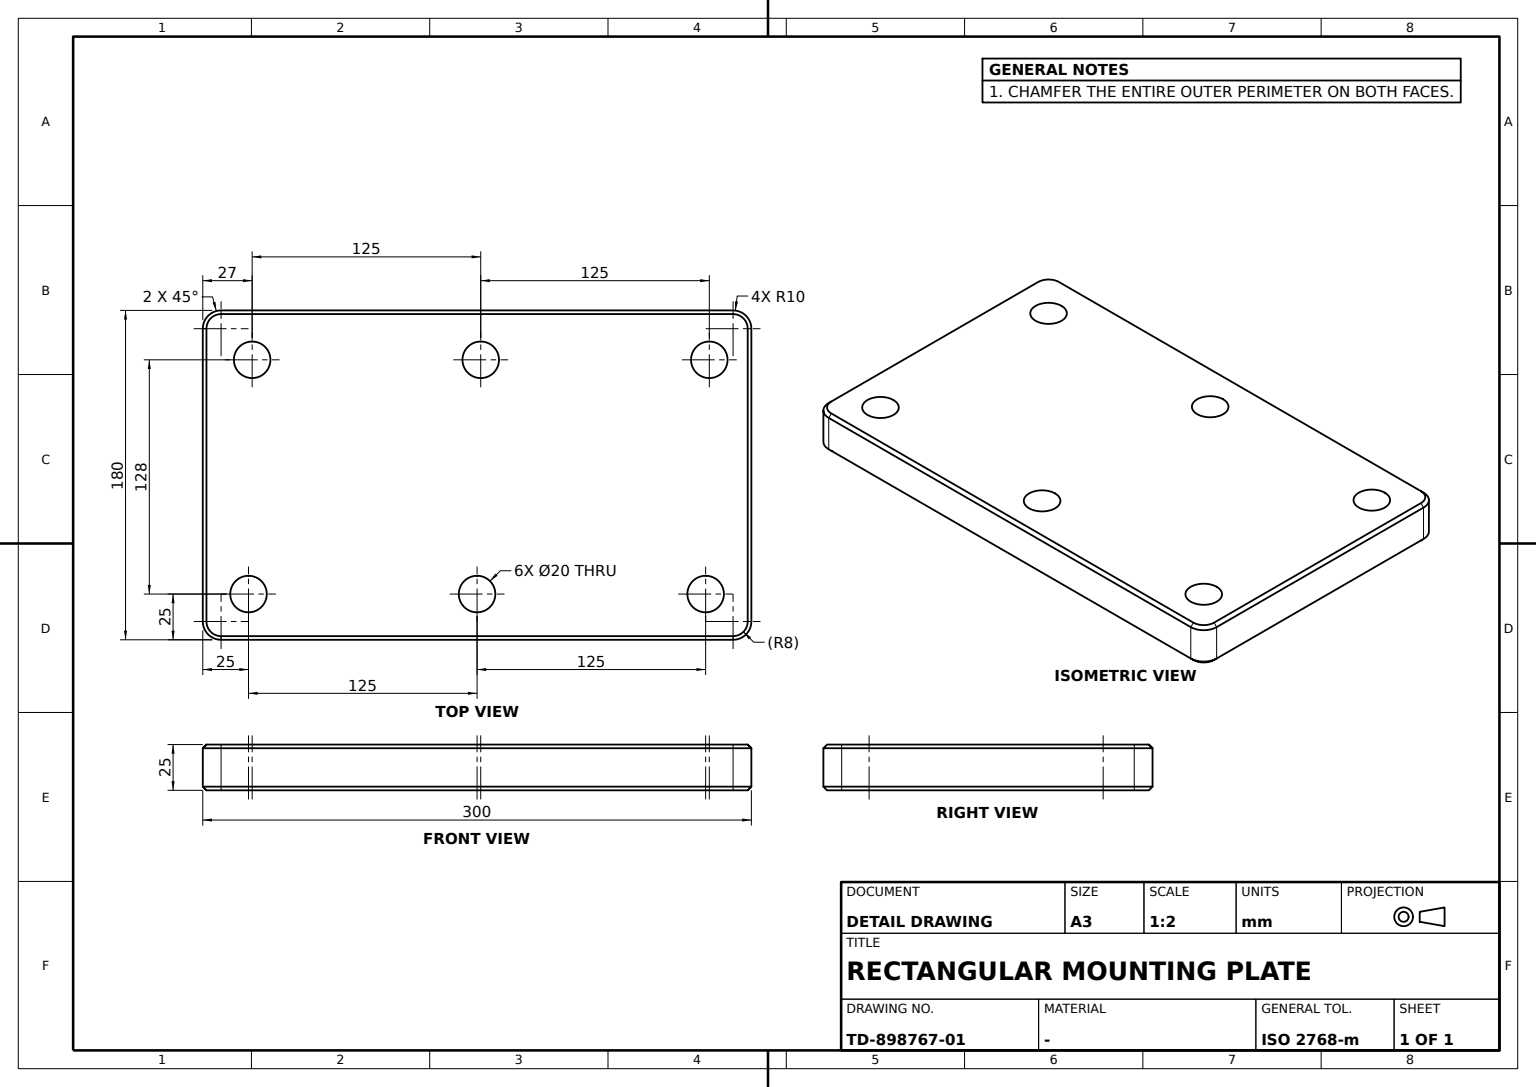
ISO-10303-21;
HEADER;
FILE_DESCRIPTION((''),'2;1');
FILE_NAME('','',(''),(''),'','','');
FILE_SCHEMA(('AUTOMOTIVE_DESIGN'));
ENDSEC;
DATA;
#1=APPLICATION_CONTEXT('');
#2=PRODUCT_CONTEXT('',#1,'mechanical');
#3=PRODUCT('','','',(#2));
#4=PRODUCT_DEFINITION_FORMATION('','',#3);
#5=PRODUCT_DEFINITION_CONTEXT('',#1,'design');
#6=PRODUCT_DEFINITION('','',#4,#5);
#7=PRODUCT_DEFINITION_SHAPE('','',#6);
#8=(LENGTH_UNIT()NAMED_UNIT(*)SI_UNIT(.MILLI.,.METRE.));
#9=(NAMED_UNIT(*)PLANE_ANGLE_UNIT()SI_UNIT($,.RADIAN.));
#10=(NAMED_UNIT(*)SI_UNIT($,.STERADIAN.)SOLID_ANGLE_UNIT());
#11=UNCERTAINTY_MEASURE_WITH_UNIT(LENGTH_MEASURE(0.005),#8,'distance_accuracy_value','');
#12=(GEOMETRIC_REPRESENTATION_CONTEXT(3)GLOBAL_UNCERTAINTY_ASSIGNED_CONTEXT((#11))GLOBAL_UNIT_ASSIGNED_CONTEXT((#8,#9,#10))REPRESENTATION_CONTEXT('',''));
#13=CARTESIAN_POINT('',(-73.,127.,12.5));
#14=VERTEX_POINT('',#13);
#15=CARTESIAN_POINT('',(-63.,127.,12.5));
#16=DIRECTION('',(0.,0.,-1.));
#17=DIRECTION('',(-1.,0.,0.));
#18=AXIS2_PLACEMENT_3D('',#15,#16,#17);
#19=CIRCLE('',#18,10.);
#20=EDGE_CURVE('',#14,#14,#19,.T.);
#21=ORIENTED_EDGE('',*,*,#20,.F.);
#22=EDGE_LOOP('',(#21));
#23=FACE_BOUND('',#22,.T.);
#24=CARTESIAN_POINT('',(-73.,127.,-12.5));
#25=VERTEX_POINT('',#24);
#26=CARTESIAN_POINT('',(-63.,127.,-12.5));
#27=AXIS2_PLACEMENT_3D('',#26,#16,#17);
#28=CIRCLE('',#27,10.);
#29=EDGE_CURVE('',#25,#25,#28,.T.);
#30=ORIENTED_EDGE('',*,*,#29,.T.);
#31=EDGE_LOOP('',(#30));
#32=FACE_BOUND('',#31,.T.);
#33=CARTESIAN_POINT('',(-63.,127.,12.4));
#34=DIRECTION('',(1.,0.,0.));
#35=AXIS2_PLACEMENT_3D('',#33,#16,#34);
#36=CYLINDRICAL_SURFACE('',#35,10.);
#37=ADVANCED_FACE('',(#23,#32),#36,.F.);
#38=CARTESIAN_POINT('',(80.,148.,-12.5));
#39=VERTEX_POINT('',#38);
#40=CARTESIAN_POINT('',(80.,150.,-10.5));
#41=VERTEX_POINT('',#40);
#42=CARTESIAN_POINT('',(80.,140.,-20.5));
#43=DIRECTION('',(0.,0.707106781,0.707106781));
#44=VECTOR('',#43,1000.);
#45=LINE('',#42,#44);
#46=EDGE_CURVE('',#39,#41,#45,.T.);
#47=ORIENTED_EDGE('',*,*,#46,.F.);
#48=CARTESIAN_POINT('',(-80.,148.,-12.5));
#49=VERTEX_POINT('',#48);
#50=CARTESIAN_POINT('',(-126.,148.,-12.5));
#51=VECTOR('',#34,1000.);
#52=LINE('',#50,#51);
#53=EDGE_CURVE('',#49,#39,#52,.T.);
#54=ORIENTED_EDGE('',*,*,#53,.F.);
#55=CARTESIAN_POINT('',(-80.,150.,-10.5));
#56=VERTEX_POINT('',#55);
#57=CARTESIAN_POINT('',(-80.,140.,-20.5));
#58=LINE('',#57,#44);
#59=EDGE_CURVE('',#49,#56,#58,.T.);
#60=ORIENTED_EDGE('',*,*,#59,.T.);
#61=CARTESIAN_POINT('',(-90.,150.,-10.5));
#62=LINE('',#61,#51);
#63=EDGE_CURVE('',#56,#41,#62,.T.);
#64=ORIENTED_EDGE('',*,*,#63,.T.);
#65=EDGE_LOOP('',(#47,#54,#60,#64));
#66=FACE_BOUND('',#65,.T.);
#67=DIRECTION('',(0.,-0.707106781,0.707106781));
#68=AXIS2_PLACEMENT_3D('',#50,#67,#34);
#69=PLANE('',#68);
#70=ADVANCED_FACE('',(#66),#69,.F.);
#71=CARTESIAN_POINT('',(-80.,150.,10.5));
#72=VERTEX_POINT('',#71);
#73=CARTESIAN_POINT('',(-80.,150.,0.));
#74=VECTOR('',#16,1000.);
#75=LINE('',#73,#74);
#76=EDGE_CURVE('',#72,#56,#75,.T.);
#77=ORIENTED_EDGE('',*,*,#76,.F.);
#78=CARTESIAN_POINT('',(80.,150.,10.5));
#79=VERTEX_POINT('',#78);
#80=CARTESIAN_POINT('',(-90.,150.,10.5));
#81=LINE('',#80,#51);
#82=EDGE_CURVE('',#72,#79,#81,.T.);
#83=ORIENTED_EDGE('',*,*,#82,.T.);
#84=CARTESIAN_POINT('',(80.,150.,0.));
#85=LINE('',#84,#74);
#86=EDGE_CURVE('',#79,#41,#85,.T.);
#87=ORIENTED_EDGE('',*,*,#86,.T.);
#88=ORIENTED_EDGE('',*,*,#63,.F.);
#89=EDGE_LOOP('',(#77,#83,#87,#88));
#90=FACE_BOUND('',#89,.T.);
#91=CARTESIAN_POINT('',(-90.,150.,0.));
#92=DIRECTION('',(0.,1.,0.));
#93=AXIS2_PLACEMENT_3D('',#91,#92,#34);
#94=PLANE('',#93);
#95=ADVANCED_FACE('',(#90),#94,.T.);
#96=CARTESIAN_POINT('',(-80.,-148.,-12.5));
#97=VERTEX_POINT('',#96);
#98=CARTESIAN_POINT('',(-80.,-150.,-10.5));
#99=VERTEX_POINT('',#98);
#100=CARTESIAN_POINT('',(-80.,-140.,-20.5));
#101=VECTOR('',#67,1000.);
#102=LINE('',#100,#101);
#103=EDGE_CURVE('',#97,#99,#102,.T.);
#104=ORIENTED_EDGE('',*,*,#103,.F.);
#105=CARTESIAN_POINT('',(80.,-148.,-12.5));
#106=VERTEX_POINT('',#105);
#107=CARTESIAN_POINT('',(126.,-148.,-12.5));
#108=VECTOR('',#17,1000.);
#109=LINE('',#107,#108);
#110=EDGE_CURVE('',#106,#97,#109,.T.);
#111=ORIENTED_EDGE('',*,*,#110,.F.);
#112=CARTESIAN_POINT('',(80.,-150.,-10.5));
#113=VERTEX_POINT('',#112);
#114=CARTESIAN_POINT('',(80.,-140.,-20.5));
#115=LINE('',#114,#101);
#116=EDGE_CURVE('',#106,#113,#115,.T.);
#117=ORIENTED_EDGE('',*,*,#116,.T.);
#118=CARTESIAN_POINT('',(90.,-150.,-10.5));
#119=LINE('',#118,#108);
#120=EDGE_CURVE('',#113,#99,#119,.T.);
#121=ORIENTED_EDGE('',*,*,#120,.T.);
#122=EDGE_LOOP('',(#104,#111,#117,#121));
#123=FACE_BOUND('',#122,.T.);
#124=AXIS2_PLACEMENT_3D('',#107,#43,#17);
#125=PLANE('',#124);
#126=ADVANCED_FACE('',(#123),#125,.F.);
#127=CARTESIAN_POINT('',(55.,0.,-12.5));
#128=VERTEX_POINT('',#127);
#129=CARTESIAN_POINT('',(65.,0.,-12.5));
#130=AXIS2_PLACEMENT_3D('',#129,#16,#17);
#131=CIRCLE('',#130,10.);
#132=EDGE_CURVE('',#128,#128,#131,.T.);
#133=ORIENTED_EDGE('',*,*,#132,.T.);
#134=EDGE_LOOP('',(#133));
#135=FACE_BOUND('',#134,.T.);
#136=CARTESIAN_POINT('',(55.,0.,12.5));
#137=VERTEX_POINT('',#136);
#138=CARTESIAN_POINT('',(65.,0.,12.5));
#139=AXIS2_PLACEMENT_3D('',#138,#16,#17);
#140=CIRCLE('',#139,10.);
#141=EDGE_CURVE('',#137,#137,#140,.T.);
#142=ORIENTED_EDGE('',*,*,#141,.F.);
#143=EDGE_LOOP('',(#142));
#144=FACE_BOUND('',#143,.T.);
#145=CARTESIAN_POINT('',(65.,0.,12.4));
#146=AXIS2_PLACEMENT_3D('',#145,#16,#34);
#147=CYLINDRICAL_SURFACE('',#146,10.);
#148=ADVANCED_FACE('',(#135,#144),#147,.F.);
#149=CARTESIAN_POINT('',(-80.,-150.,10.5));
#150=VERTEX_POINT('',#149);
#151=CARTESIAN_POINT('',(-90.,-140.,10.5));
#152=VERTEX_POINT('',#151);
#153=CARTESIAN_POINT('',(-80.,-140.,10.5));
#154=AXIS2_PLACEMENT_3D('',#153,#16,#17);
#155=CIRCLE('',#154,10.);
#156=EDGE_CURVE('',#150,#152,#155,.T.);
#157=ORIENTED_EDGE('',*,*,#156,.F.);
#158=CARTESIAN_POINT('',(-80.,-148.,12.5));
#159=VERTEX_POINT('',#158);
#160=CARTESIAN_POINT('',(-80.,-140.,20.5));
#161=DIRECTION('',(0.,-0.707106781,-0.707106781));
#162=VECTOR('',#161,1000.);
#163=LINE('',#160,#162);
#164=EDGE_CURVE('',#159,#150,#163,.T.);
#165=ORIENTED_EDGE('',*,*,#164,.F.);
#166=CARTESIAN_POINT('',(-88.,-140.,12.5));
#167=VERTEX_POINT('',#166);
#168=CARTESIAN_POINT('',(-80.,-140.,12.5));
#169=AXIS2_PLACEMENT_3D('',#168,#16,#17);
#170=CIRCLE('',#169,8.);
#171=EDGE_CURVE('',#159,#167,#170,.T.);
#172=ORIENTED_EDGE('',*,*,#171,.T.);
#173=DIRECTION('',(-0.707106781,0.,-0.707106781));
#174=VECTOR('',#173,1000.);
#175=LINE('',#160,#174);
#176=EDGE_CURVE('',#167,#152,#175,.T.);
#177=ORIENTED_EDGE('',*,*,#176,.T.);
#178=EDGE_LOOP('',(#157,#165,#172,#177));
#179=FACE_BOUND('',#178,.T.);
#180=DIRECTION('',(0.459989449,-0.887924381,0.));
#181=AXIS2_PLACEMENT_3D('',#160,#16,#180);
#182=CONICAL_SURFACE('',#181,0.,0.785398163);
#183=ADVANCED_FACE('',(#179),#182,.T.);
#184=CARTESIAN_POINT('',(-80.,-150.,0.));
#185=LINE('',#184,#74);
#186=EDGE_CURVE('',#150,#99,#185,.T.);
#187=ORIENTED_EDGE('',*,*,#186,.T.);
#188=ORIENTED_EDGE('',*,*,#120,.F.);
#189=CARTESIAN_POINT('',(80.,-150.,10.5));
#190=VERTEX_POINT('',#189);
#191=CARTESIAN_POINT('',(80.,-150.,0.));
#192=LINE('',#191,#74);
#193=EDGE_CURVE('',#190,#113,#192,.T.);
#194=ORIENTED_EDGE('',*,*,#193,.F.);
#195=CARTESIAN_POINT('',(90.,-150.,10.5));
#196=LINE('',#195,#108);
#197=EDGE_CURVE('',#190,#150,#196,.T.);
#198=ORIENTED_EDGE('',*,*,#197,.T.);
#199=EDGE_LOOP('',(#187,#188,#194,#198));
#200=FACE_BOUND('',#199,.T.);
#201=CARTESIAN_POINT('',(90.,-150.,0.));
#202=DIRECTION('',(0.,-1.,0.));
#203=AXIS2_PLACEMENT_3D('',#201,#202,#17);
#204=PLANE('',#203);
#205=ADVANCED_FACE('',(#200),#204,.T.);
#206=CARTESIAN_POINT('',(90.,140.,10.5));
#207=VERTEX_POINT('',#206);
#208=CARTESIAN_POINT('',(90.,140.,-10.5));
#209=VERTEX_POINT('',#208);
#210=CARTESIAN_POINT('',(90.,140.,0.));
#211=LINE('',#210,#74);
#212=EDGE_CURVE('',#207,#209,#211,.T.);
#213=ORIENTED_EDGE('',*,*,#212,.F.);
#214=CARTESIAN_POINT('',(90.,-140.,10.5));
#215=VERTEX_POINT('',#214);
#216=CARTESIAN_POINT('',(90.,-210.,10.5));
#217=VECTOR('',#92,1000.);
#218=LINE('',#216,#217);
#219=EDGE_CURVE('',#215,#207,#218,.T.);
#220=ORIENTED_EDGE('',*,*,#219,.F.);
#221=CARTESIAN_POINT('',(90.,-140.,-10.5));
#222=VERTEX_POINT('',#221);
#223=CARTESIAN_POINT('',(90.,-140.,0.));
#224=LINE('',#223,#74);
#225=EDGE_CURVE('',#215,#222,#224,.T.);
#226=ORIENTED_EDGE('',*,*,#225,.T.);
#227=CARTESIAN_POINT('',(90.,-210.,-10.5));
#228=LINE('',#227,#217);
#229=EDGE_CURVE('',#222,#209,#228,.T.);
#230=ORIENTED_EDGE('',*,*,#229,.T.);
#231=EDGE_LOOP('',(#213,#220,#226,#230));
#232=FACE_BOUND('',#231,.T.);
#233=AXIS2_PLACEMENT_3D('',#201,#17,#92);
#234=PLANE('',#233);
#235=ADVANCED_FACE('',(#232),#234,.F.);
#236=CARTESIAN_POINT('',(-90.,140.,-10.5));
#237=VERTEX_POINT('',#236);
#238=CARTESIAN_POINT('',(-90.,-140.,-10.5));
#239=VERTEX_POINT('',#238);
#240=CARTESIAN_POINT('',(-90.,210.,-10.5));
#241=VECTOR('',#202,1000.);
#242=LINE('',#240,#241);
#243=EDGE_CURVE('',#237,#239,#242,.T.);
#244=ORIENTED_EDGE('',*,*,#243,.F.);
#245=CARTESIAN_POINT('',(-88.,140.,-12.5));
#246=VERTEX_POINT('',#245);
#247=DIRECTION('',(-0.707106781,0.,0.707106781));
#248=VECTOR('',#247,1000.);
#249=LINE('',#57,#248);
#250=EDGE_CURVE('',#246,#237,#249,.T.);
#251=ORIENTED_EDGE('',*,*,#250,.F.);
#252=CARTESIAN_POINT('',(-88.,-140.,-12.5));
#253=VERTEX_POINT('',#252);
#254=CARTESIAN_POINT('',(-88.,210.,-12.5));
#255=LINE('',#254,#241);
#256=EDGE_CURVE('',#246,#253,#255,.T.);
#257=ORIENTED_EDGE('',*,*,#256,.T.);
#258=LINE('',#100,#248);
#259=EDGE_CURVE('',#253,#239,#258,.T.);
#260=ORIENTED_EDGE('',*,*,#259,.T.);
#261=EDGE_LOOP('',(#244,#251,#257,#260));
#262=FACE_BOUND('',#261,.T.);
#263=AXIS2_PLACEMENT_3D('',#254,#173,#202);
#264=PLANE('',#263);
#265=ADVANCED_FACE('',(#262),#264,.T.);
#266=CARTESIAN_POINT('',(88.,-140.,12.5));
#267=VERTEX_POINT('',#266);
#268=CARTESIAN_POINT('',(80.,-148.,12.5));
#269=VERTEX_POINT('',#268);
#270=CARTESIAN_POINT('',(80.,-140.,12.5));
#271=AXIS2_PLACEMENT_3D('',#270,#16,#17);
#272=CIRCLE('',#271,8.);
#273=EDGE_CURVE('',#267,#269,#272,.T.);
#274=ORIENTED_EDGE('',*,*,#273,.T.);
#275=CARTESIAN_POINT('',(80.,-140.,20.5));
#276=LINE('',#275,#162);
#277=EDGE_CURVE('',#269,#190,#276,.T.);
#278=ORIENTED_EDGE('',*,*,#277,.T.);
#279=CARTESIAN_POINT('',(80.,-140.,10.5));
#280=AXIS2_PLACEMENT_3D('',#279,#16,#92);
#281=CIRCLE('',#280,10.);
#282=EDGE_CURVE('',#215,#190,#281,.T.);
#283=ORIENTED_EDGE('',*,*,#282,.F.);
#284=DIRECTION('',(0.707106781,0.,-0.707106781));
#285=VECTOR('',#284,1000.);
#286=LINE('',#275,#285);
#287=EDGE_CURVE('',#267,#215,#286,.T.);
#288=ORIENTED_EDGE('',*,*,#287,.F.);
#289=EDGE_LOOP('',(#274,#278,#283,#288));
#290=FACE_BOUND('',#289,.T.);
#291=DIRECTION('',(0.887924381,0.459989449,0.));
#292=AXIS2_PLACEMENT_3D('',#275,#16,#291);
#293=CONICAL_SURFACE('',#292,0.,0.785398163);
#294=ADVANCED_FACE('',(#290),#293,.T.);
#295=ORIENTED_EDGE('',*,*,#116,.F.);
#296=CARTESIAN_POINT('',(88.,-140.,-12.5));
#297=VERTEX_POINT('',#296);
#298=CARTESIAN_POINT('',(80.,-140.,-12.5));
#299=AXIS2_PLACEMENT_3D('',#298,#16,#17);
#300=CIRCLE('',#299,8.);
#301=EDGE_CURVE('',#297,#106,#300,.T.);
#302=ORIENTED_EDGE('',*,*,#301,.F.);
#303=DIRECTION('',(0.707106781,0.,0.707106781));
#304=VECTOR('',#303,1000.);
#305=LINE('',#114,#304);
#306=EDGE_CURVE('',#297,#222,#305,.T.);
#307=ORIENTED_EDGE('',*,*,#306,.T.);
#308=CARTESIAN_POINT('',(80.,-140.,-10.5));
#309=DIRECTION('',(0.,0.,1.));
#310=AXIS2_PLACEMENT_3D('',#308,#309,#202);
#311=CIRCLE('',#310,10.);
#312=EDGE_CURVE('',#222,#113,#311,.F.);
#313=ORIENTED_EDGE('',*,*,#312,.T.);
#314=EDGE_LOOP('',(#295,#302,#307,#313));
#315=FACE_BOUND('',#314,.T.);
#316=DIRECTION('',(-0.887924381,-0.459989449,0.));
#317=AXIS2_PLACEMENT_3D('',#114,#309,#316);
#318=CONICAL_SURFACE('',#317,0.,0.785398163);
#319=ADVANCED_FACE('',(#315),#318,.T.);
#320=CARTESIAN_POINT('',(-73.,-123.,-12.5));
#321=VERTEX_POINT('',#320);
#322=CARTESIAN_POINT('',(-63.,-123.,-12.5));
#323=AXIS2_PLACEMENT_3D('',#322,#16,#17);
#324=CIRCLE('',#323,10.);
#325=EDGE_CURVE('',#321,#321,#324,.T.);
#326=ORIENTED_EDGE('',*,*,#325,.T.);
#327=EDGE_LOOP('',(#326));
#328=FACE_BOUND('',#327,.T.);
#329=CARTESIAN_POINT('',(-73.,-123.,12.5));
#330=VERTEX_POINT('',#329);
#331=CARTESIAN_POINT('',(-63.,-123.,12.5));
#332=AXIS2_PLACEMENT_3D('',#331,#16,#17);
#333=CIRCLE('',#332,10.);
#334=EDGE_CURVE('',#330,#330,#333,.T.);
#335=ORIENTED_EDGE('',*,*,#334,.F.);
#336=EDGE_LOOP('',(#335));
#337=FACE_BOUND('',#336,.T.);
#338=CARTESIAN_POINT('',(-63.,-123.,12.4));
#339=AXIS2_PLACEMENT_3D('',#338,#16,#34);
#340=CYLINDRICAL_SURFACE('',#339,10.);
#341=ADVANCED_FACE('',(#328,#337),#340,.F.);
#342=ORIENTED_EDGE('',*,*,#59,.F.);
#343=CARTESIAN_POINT('',(-80.,140.,-12.5));
#344=AXIS2_PLACEMENT_3D('',#343,#16,#17);
#345=CIRCLE('',#344,8.);
#346=EDGE_CURVE('',#246,#49,#345,.T.);
#347=ORIENTED_EDGE('',*,*,#346,.F.);
#348=ORIENTED_EDGE('',*,*,#250,.T.);
#349=CARTESIAN_POINT('',(-80.,140.,-10.5));
#350=AXIS2_PLACEMENT_3D('',#349,#309,#202);
#351=CIRCLE('',#350,10.);
#352=EDGE_CURVE('',#237,#56,#351,.F.);
#353=ORIENTED_EDGE('',*,*,#352,.T.);
#354=EDGE_LOOP('',(#342,#347,#348,#353));
#355=FACE_BOUND('',#354,.T.);
#356=AXIS2_PLACEMENT_3D('',#57,#309,#291);
#357=CONICAL_SURFACE('',#356,0.,0.785398163);
#358=ADVANCED_FACE('',(#355),#357,.T.);
#359=ORIENTED_EDGE('',*,*,#259,.F.);
#360=CARTESIAN_POINT('',(-80.,-140.,-12.5));
#361=AXIS2_PLACEMENT_3D('',#360,#16,#17);
#362=CIRCLE('',#361,8.);
#363=EDGE_CURVE('',#97,#253,#362,.T.);
#364=ORIENTED_EDGE('',*,*,#363,.F.);
#365=ORIENTED_EDGE('',*,*,#103,.T.);
#366=CARTESIAN_POINT('',(-80.,-140.,-10.5));
#367=AXIS2_PLACEMENT_3D('',#366,#309,#34);
#368=CIRCLE('',#367,10.);
#369=EDGE_CURVE('',#99,#239,#368,.F.);
#370=ORIENTED_EDGE('',*,*,#369,.T.);
#371=EDGE_LOOP('',(#359,#364,#365,#370));
#372=FACE_BOUND('',#371,.T.);
#373=DIRECTION('',(-0.459989449,0.887924381,0.));
#374=AXIS2_PLACEMENT_3D('',#100,#309,#373);
#375=CONICAL_SURFACE('',#374,0.,0.785398163);
#376=ADVANCED_FACE('',(#372),#375,.T.);
#377=CARTESIAN_POINT('',(0.,-148.,12.5));
#378=LINE('',#377,#108);
#379=EDGE_CURVE('',#269,#159,#378,.T.);
#380=ORIENTED_EDGE('',*,*,#379,.T.);
#381=ORIENTED_EDGE('',*,*,#164,.T.);
#382=ORIENTED_EDGE('',*,*,#197,.F.);
#383=ORIENTED_EDGE('',*,*,#277,.F.);
#384=EDGE_LOOP('',(#380,#381,#382,#383));
#385=FACE_BOUND('',#384,.T.);
#386=CARTESIAN_POINT('',(126.,-148.,12.5));
#387=AXIS2_PLACEMENT_3D('',#386,#67,#17);
#388=PLANE('',#387);
#389=ADVANCED_FACE('',(#385),#388,.T.);
#390=ORIENTED_EDGE('',*,*,#193,.T.);
#391=ORIENTED_EDGE('',*,*,#312,.F.);
#392=ORIENTED_EDGE('',*,*,#225,.F.);
#393=ORIENTED_EDGE('',*,*,#282,.T.);
#394=EDGE_LOOP('',(#390,#391,#392,#393));
#395=FACE_BOUND('',#394,.T.);
#396=CARTESIAN_POINT('',(80.,-140.,0.));
#397=AXIS2_PLACEMENT_3D('',#396,#16,#202);
#398=CYLINDRICAL_SURFACE('',#397,10.);
#399=ADVANCED_FACE('',(#395),#398,.T.);
#400=ORIENTED_EDGE('',*,*,#186,.F.);
#401=ORIENTED_EDGE('',*,*,#156,.T.);
#402=CARTESIAN_POINT('',(-90.,-140.,0.));
#403=LINE('',#402,#74);
#404=EDGE_CURVE('',#152,#239,#403,.T.);
#405=ORIENTED_EDGE('',*,*,#404,.T.);
#406=ORIENTED_EDGE('',*,*,#369,.F.);
#407=EDGE_LOOP('',(#400,#401,#405,#406));
#408=FACE_BOUND('',#407,.T.);
#409=CARTESIAN_POINT('',(-80.,-140.,0.));
#410=AXIS2_PLACEMENT_3D('',#409,#16,#17);
#411=CYLINDRICAL_SURFACE('',#410,10.);
#412=ADVANCED_FACE('',(#408),#411,.T.);
#413=CARTESIAN_POINT('',(-73.,2.,12.5));
#414=VERTEX_POINT('',#413);
#415=CARTESIAN_POINT('',(-63.,2.,12.5));
#416=AXIS2_PLACEMENT_3D('',#415,#16,#17);
#417=CIRCLE('',#416,10.);
#418=EDGE_CURVE('',#414,#414,#417,.T.);
#419=ORIENTED_EDGE('',*,*,#418,.F.);
#420=EDGE_LOOP('',(#419));
#421=FACE_BOUND('',#420,.T.);
#422=CARTESIAN_POINT('',(-73.,2.,-12.5));
#423=VERTEX_POINT('',#422);
#424=CARTESIAN_POINT('',(-63.,2.,-12.5));
#425=AXIS2_PLACEMENT_3D('',#424,#16,#17);
#426=CIRCLE('',#425,10.);
#427=EDGE_CURVE('',#423,#423,#426,.T.);
#428=ORIENTED_EDGE('',*,*,#427,.T.);
#429=EDGE_LOOP('',(#428));
#430=FACE_BOUND('',#429,.T.);
#431=CARTESIAN_POINT('',(-63.,2.,12.4));
#432=AXIS2_PLACEMENT_3D('',#431,#16,#34);
#433=CYLINDRICAL_SURFACE('',#432,10.);
#434=ADVANCED_FACE('',(#421,#430),#433,.F.);
#435=ORIENTED_EDGE('',*,*,#352,.F.);
#436=CARTESIAN_POINT('',(-90.,140.,10.5));
#437=VERTEX_POINT('',#436);
#438=CARTESIAN_POINT('',(-90.,140.,0.));
#439=LINE('',#438,#74);
#440=EDGE_CURVE('',#437,#237,#439,.T.);
#441=ORIENTED_EDGE('',*,*,#440,.F.);
#442=CARTESIAN_POINT('',(-80.,140.,10.5));
#443=AXIS2_PLACEMENT_3D('',#442,#16,#92);
#444=CIRCLE('',#443,10.);
#445=EDGE_CURVE('',#437,#72,#444,.T.);
#446=ORIENTED_EDGE('',*,*,#445,.T.);
#447=ORIENTED_EDGE('',*,*,#76,.T.);
#448=EDGE_LOOP('',(#435,#441,#446,#447));
#449=FACE_BOUND('',#448,.T.);
#450=CARTESIAN_POINT('',(-80.,140.,0.));
#451=AXIS2_PLACEMENT_3D('',#450,#16,#92);
#452=CYLINDRICAL_SURFACE('',#451,10.);
#453=ADVANCED_FACE('',(#449),#452,.T.);
#454=CARTESIAN_POINT('',(88.,140.,-12.5));
#455=VERTEX_POINT('',#454);
#456=LINE('',#42,#304);
#457=EDGE_CURVE('',#455,#209,#456,.T.);
#458=ORIENTED_EDGE('',*,*,#457,.F.);
#459=CARTESIAN_POINT('',(80.,140.,-12.5));
#460=AXIS2_PLACEMENT_3D('',#459,#16,#17);
#461=CIRCLE('',#460,8.);
#462=EDGE_CURVE('',#39,#455,#461,.T.);
#463=ORIENTED_EDGE('',*,*,#462,.F.);
#464=ORIENTED_EDGE('',*,*,#46,.T.);
#465=CARTESIAN_POINT('',(80.,140.,-10.5));
#466=AXIS2_PLACEMENT_3D('',#465,#309,#34);
#467=CIRCLE('',#466,10.);
#468=EDGE_CURVE('',#41,#209,#467,.F.);
#469=ORIENTED_EDGE('',*,*,#468,.T.);
#470=EDGE_LOOP('',(#458,#463,#464,#469));
#471=FACE_BOUND('',#470,.T.);
#472=AXIS2_PLACEMENT_3D('',#42,#309,#180);
#473=CONICAL_SURFACE('',#472,0.,0.785398163);
#474=ADVANCED_FACE('',(#471),#473,.T.);
#475=ORIENTED_EDGE('',*,*,#445,.F.);
#476=CARTESIAN_POINT('',(-88.,140.,12.5));
#477=VERTEX_POINT('',#476);
#478=CARTESIAN_POINT('',(-80.,140.,20.5));
#479=LINE('',#478,#174);
#480=EDGE_CURVE('',#477,#437,#479,.T.);
#481=ORIENTED_EDGE('',*,*,#480,.F.);
#482=CARTESIAN_POINT('',(-80.,148.,12.5));
#483=VERTEX_POINT('',#482);
#484=CARTESIAN_POINT('',(-80.,140.,12.5));
#485=AXIS2_PLACEMENT_3D('',#484,#16,#17);
#486=CIRCLE('',#485,8.);
#487=EDGE_CURVE('',#477,#483,#486,.T.);
#488=ORIENTED_EDGE('',*,*,#487,.T.);
#489=DIRECTION('',(0.,0.707106781,-0.707106781));
#490=VECTOR('',#489,1000.);
#491=LINE('',#478,#490);
#492=EDGE_CURVE('',#483,#72,#491,.T.);
#493=ORIENTED_EDGE('',*,*,#492,.T.);
#494=EDGE_LOOP('',(#475,#481,#488,#493));
#495=FACE_BOUND('',#494,.T.);
#496=AXIS2_PLACEMENT_3D('',#478,#16,#316);
#497=CONICAL_SURFACE('',#496,0.,0.785398163);
#498=ADVANCED_FACE('',(#495),#497,.T.);
#499=CARTESIAN_POINT('',(80.,148.,12.5));
#500=VERTEX_POINT('',#499);
#501=CARTESIAN_POINT('',(80.,140.,20.5));
#502=LINE('',#501,#490);
#503=EDGE_CURVE('',#500,#79,#502,.T.);
#504=ORIENTED_EDGE('',*,*,#503,.T.);
#505=ORIENTED_EDGE('',*,*,#82,.F.);
#506=ORIENTED_EDGE('',*,*,#492,.F.);
#507=CARTESIAN_POINT('',(0.,148.,12.5));
#508=LINE('',#507,#51);
#509=EDGE_CURVE('',#483,#500,#508,.T.);
#510=ORIENTED_EDGE('',*,*,#509,.T.);
#511=EDGE_LOOP('',(#504,#505,#506,#510));
#512=FACE_BOUND('',#511,.T.);
#513=CARTESIAN_POINT('',(-126.,148.,12.5));
#514=AXIS2_PLACEMENT_3D('',#513,#43,#34);
#515=PLANE('',#514);
#516=ADVANCED_FACE('',(#512),#515,.T.);
#517=CARTESIAN_POINT('',(88.,140.,12.5));
#518=VERTEX_POINT('',#517);
#519=CARTESIAN_POINT('',(88.,0.,12.5));
#520=LINE('',#519,#217);
#521=EDGE_CURVE('',#267,#518,#520,.T.);
#522=ORIENTED_EDGE('',*,*,#521,.F.);
#523=ORIENTED_EDGE('',*,*,#287,.T.);
#524=ORIENTED_EDGE('',*,*,#219,.T.);
#525=LINE('',#501,#285);
#526=EDGE_CURVE('',#518,#207,#525,.T.);
#527=ORIENTED_EDGE('',*,*,#526,.F.);
#528=EDGE_LOOP('',(#522,#523,#524,#527));
#529=FACE_BOUND('',#528,.T.);
#530=CARTESIAN_POINT('',(88.,-210.,12.5));
#531=AXIS2_PLACEMENT_3D('',#530,#173,#92);
#532=PLANE('',#531);
#533=ADVANCED_FACE('',(#529),#532,.F.);
#534=ORIENTED_EDGE('',*,*,#229,.F.);
#535=ORIENTED_EDGE('',*,*,#306,.F.);
#536=CARTESIAN_POINT('',(88.,-210.,-12.5));
#537=LINE('',#536,#217);
#538=EDGE_CURVE('',#297,#455,#537,.T.);
#539=ORIENTED_EDGE('',*,*,#538,.T.);
#540=ORIENTED_EDGE('',*,*,#457,.T.);
#541=EDGE_LOOP('',(#534,#535,#539,#540));
#542=FACE_BOUND('',#541,.T.);
#543=AXIS2_PLACEMENT_3D('',#536,#284,#92);
#544=PLANE('',#543);
#545=ADVANCED_FACE('',(#542),#544,.T.);
#546=CARTESIAN_POINT('',(55.,125.,12.5));
#547=VERTEX_POINT('',#546);
#548=CARTESIAN_POINT('',(65.,125.,12.5));
#549=AXIS2_PLACEMENT_3D('',#548,#16,#17);
#550=CIRCLE('',#549,10.);
#551=EDGE_CURVE('',#547,#547,#550,.T.);
#552=ORIENTED_EDGE('',*,*,#551,.T.);
#553=EDGE_LOOP('',(#552));
#554=FACE_BOUND('',#553,.T.);
#555=ORIENTED_EDGE('',*,*,#334,.T.);
#556=EDGE_LOOP('',(#555));
#557=FACE_BOUND('',#556,.T.);
#558=CARTESIAN_POINT('',(55.,-125.,12.5));
#559=VERTEX_POINT('',#558);
#560=CARTESIAN_POINT('',(65.,-125.,12.5));
#561=AXIS2_PLACEMENT_3D('',#560,#16,#17);
#562=CIRCLE('',#561,10.);
#563=EDGE_CURVE('',#559,#559,#562,.T.);
#564=ORIENTED_EDGE('',*,*,#563,.T.);
#565=EDGE_LOOP('',(#564));
#566=FACE_BOUND('',#565,.T.);
#567=ORIENTED_EDGE('',*,*,#141,.T.);
#568=EDGE_LOOP('',(#567));
#569=FACE_BOUND('',#568,.T.);
#570=ORIENTED_EDGE('',*,*,#509,.F.);
#571=ORIENTED_EDGE('',*,*,#487,.F.);
#572=CARTESIAN_POINT('',(-88.,0.,12.5));
#573=LINE('',#572,#241);
#574=EDGE_CURVE('',#477,#167,#573,.T.);
#575=ORIENTED_EDGE('',*,*,#574,.T.);
#576=ORIENTED_EDGE('',*,*,#171,.F.);
#577=ORIENTED_EDGE('',*,*,#379,.F.);
#578=ORIENTED_EDGE('',*,*,#273,.F.);
#579=ORIENTED_EDGE('',*,*,#521,.T.);
#580=CARTESIAN_POINT('',(80.,140.,12.5));
#581=AXIS2_PLACEMENT_3D('',#580,#16,#17);
#582=CIRCLE('',#581,8.);
#583=EDGE_CURVE('',#500,#518,#582,.T.);
#584=ORIENTED_EDGE('',*,*,#583,.F.);
#585=EDGE_LOOP('',(#570,#571,#575,#576,#577,#578,#579,#584));
#586=FACE_BOUND('',#585,.T.);
#587=ORIENTED_EDGE('',*,*,#418,.T.);
#588=EDGE_LOOP('',(#587));
#589=FACE_BOUND('',#588,.T.);
#590=ORIENTED_EDGE('',*,*,#20,.T.);
#591=EDGE_LOOP('',(#590));
#592=FACE_BOUND('',#591,.T.);
#593=CARTESIAN_POINT('',(0.,0.,12.5));
#594=AXIS2_PLACEMENT_3D('',#593,#16,#92);
#595=PLANE('',#594);
#596=ADVANCED_FACE('',(#554,#557,#566,#569,#586,#589,#592),#595,.F.);
#597=CARTESIAN_POINT('',(80.,140.,10.5));
#598=AXIS2_PLACEMENT_3D('',#597,#16,#17);
#599=CIRCLE('',#598,10.);
#600=EDGE_CURVE('',#79,#207,#599,.T.);
#601=ORIENTED_EDGE('',*,*,#600,.T.);
#602=ORIENTED_EDGE('',*,*,#212,.T.);
#603=ORIENTED_EDGE('',*,*,#468,.F.);
#604=ORIENTED_EDGE('',*,*,#86,.F.);
#605=EDGE_LOOP('',(#601,#602,#603,#604));
#606=FACE_BOUND('',#605,.T.);
#607=CARTESIAN_POINT('',(80.,140.,0.));
#608=AXIS2_PLACEMENT_3D('',#607,#16,#34);
#609=CYLINDRICAL_SURFACE('',#608,10.);
#610=ADVANCED_FACE('',(#606),#609,.T.);
#611=ORIENTED_EDGE('',*,*,#503,.F.);
#612=ORIENTED_EDGE('',*,*,#583,.T.);
#613=ORIENTED_EDGE('',*,*,#526,.T.);
#614=ORIENTED_EDGE('',*,*,#600,.F.);
#615=EDGE_LOOP('',(#611,#612,#613,#614));
#616=FACE_BOUND('',#615,.T.);
#617=AXIS2_PLACEMENT_3D('',#501,#16,#373);
#618=CONICAL_SURFACE('',#617,0.,0.785398163);
#619=ADVANCED_FACE('',(#616),#618,.T.);
#620=ORIENTED_EDGE('',*,*,#243,.T.);
#621=ORIENTED_EDGE('',*,*,#404,.F.);
#622=CARTESIAN_POINT('',(-90.,210.,10.5));
#623=LINE('',#622,#241);
#624=EDGE_CURVE('',#437,#152,#623,.T.);
#625=ORIENTED_EDGE('',*,*,#624,.F.);
#626=ORIENTED_EDGE('',*,*,#440,.T.);
#627=EDGE_LOOP('',(#620,#621,#625,#626));
#628=FACE_BOUND('',#627,.T.);
#629=AXIS2_PLACEMENT_3D('',#91,#34,#202);
#630=PLANE('',#629);
#631=ADVANCED_FACE('',(#628),#630,.F.);
#632=ORIENTED_EDGE('',*,*,#563,.F.);
#633=EDGE_LOOP('',(#632));
#634=FACE_BOUND('',#633,.T.);
#635=CARTESIAN_POINT('',(55.,-125.,-12.5));
#636=VERTEX_POINT('',#635);
#637=CARTESIAN_POINT('',(65.,-125.,-12.5));
#638=AXIS2_PLACEMENT_3D('',#637,#16,#17);
#639=CIRCLE('',#638,10.);
#640=EDGE_CURVE('',#636,#636,#639,.T.);
#641=ORIENTED_EDGE('',*,*,#640,.T.);
#642=EDGE_LOOP('',(#641));
#643=FACE_BOUND('',#642,.T.);
#644=CARTESIAN_POINT('',(65.,-125.,12.4));
#645=AXIS2_PLACEMENT_3D('',#644,#16,#34);
#646=CYLINDRICAL_SURFACE('',#645,10.);
#647=ADVANCED_FACE('',(#634,#643),#646,.F.);
#648=ORIENTED_EDGE('',*,*,#574,.F.);
#649=ORIENTED_EDGE('',*,*,#480,.T.);
#650=ORIENTED_EDGE('',*,*,#624,.T.);
#651=ORIENTED_EDGE('',*,*,#176,.F.);
#652=EDGE_LOOP('',(#648,#649,#650,#651));
#653=FACE_BOUND('',#652,.T.);
#654=CARTESIAN_POINT('',(-88.,210.,12.5));
#655=AXIS2_PLACEMENT_3D('',#654,#284,#202);
#656=PLANE('',#655);
#657=ADVANCED_FACE('',(#653),#656,.F.);
#658=CARTESIAN_POINT('',(55.,125.,-12.5));
#659=VERTEX_POINT('',#658);
#660=CARTESIAN_POINT('',(65.,125.,-12.5));
#661=AXIS2_PLACEMENT_3D('',#660,#16,#17);
#662=CIRCLE('',#661,10.);
#663=EDGE_CURVE('',#659,#659,#662,.T.);
#664=ORIENTED_EDGE('',*,*,#663,.T.);
#665=EDGE_LOOP('',(#664));
#666=FACE_BOUND('',#665,.T.);
#667=ORIENTED_EDGE('',*,*,#551,.F.);
#668=EDGE_LOOP('',(#667));
#669=FACE_BOUND('',#668,.T.);
#670=CARTESIAN_POINT('',(65.,125.,12.4));
#671=AXIS2_PLACEMENT_3D('',#670,#16,#34);
#672=CYLINDRICAL_SURFACE('',#671,10.);
#673=ADVANCED_FACE('',(#666,#669),#672,.F.);
#674=ORIENTED_EDGE('',*,*,#663,.F.);
#675=EDGE_LOOP('',(#674));
#676=FACE_BOUND('',#675,.T.);
#677=ORIENTED_EDGE('',*,*,#640,.F.);
#678=EDGE_LOOP('',(#677));
#679=FACE_BOUND('',#678,.T.);
#680=ORIENTED_EDGE('',*,*,#132,.F.);
#681=EDGE_LOOP('',(#680));
#682=FACE_BOUND('',#681,.T.);
#683=ORIENTED_EDGE('',*,*,#29,.F.);
#684=EDGE_LOOP('',(#683));
#685=FACE_BOUND('',#684,.T.);
#686=ORIENTED_EDGE('',*,*,#256,.F.);
#687=ORIENTED_EDGE('',*,*,#346,.T.);
#688=ORIENTED_EDGE('',*,*,#53,.T.);
#689=ORIENTED_EDGE('',*,*,#462,.T.);
#690=ORIENTED_EDGE('',*,*,#538,.F.);
#691=ORIENTED_EDGE('',*,*,#301,.T.);
#692=ORIENTED_EDGE('',*,*,#110,.T.);
#693=ORIENTED_EDGE('',*,*,#363,.T.);
#694=EDGE_LOOP('',(#686,#687,#688,#689,#690,#691,#692,#693));
#695=FACE_BOUND('',#694,.T.);
#696=ORIENTED_EDGE('',*,*,#427,.F.);
#697=EDGE_LOOP('',(#696));
#698=FACE_BOUND('',#697,.T.);
#699=ORIENTED_EDGE('',*,*,#325,.F.);
#700=EDGE_LOOP('',(#699));
#701=FACE_BOUND('',#700,.T.);
#702=CARTESIAN_POINT('',(0.,0.,-12.5));
#703=AXIS2_PLACEMENT_3D('',#702,#16,#92);
#704=PLANE('',#703);
#705=ADVANCED_FACE('',(#676,#679,#682,#685,#695,#698,#701),#704,.T.);
#706=CLOSED_SHELL('',(#37,#70,#95,#126,#148,#183,#205,#235,#265,#294,#319,#341,#358,#376,#389,#399,#412,#434,#453,#474,#498,#516,#533,#545,#596,#610,#619,#631,#647,#657,#673,#705));
#707=MANIFOLD_SOLID_BREP('',#706);
#708=ADVANCED_BREP_SHAPE_REPRESENTATION('',(#707),#12);
#709=SHAPE_DEFINITION_REPRESENTATION(#7,#708);
ENDSEC;
END-ISO-10303-21;
